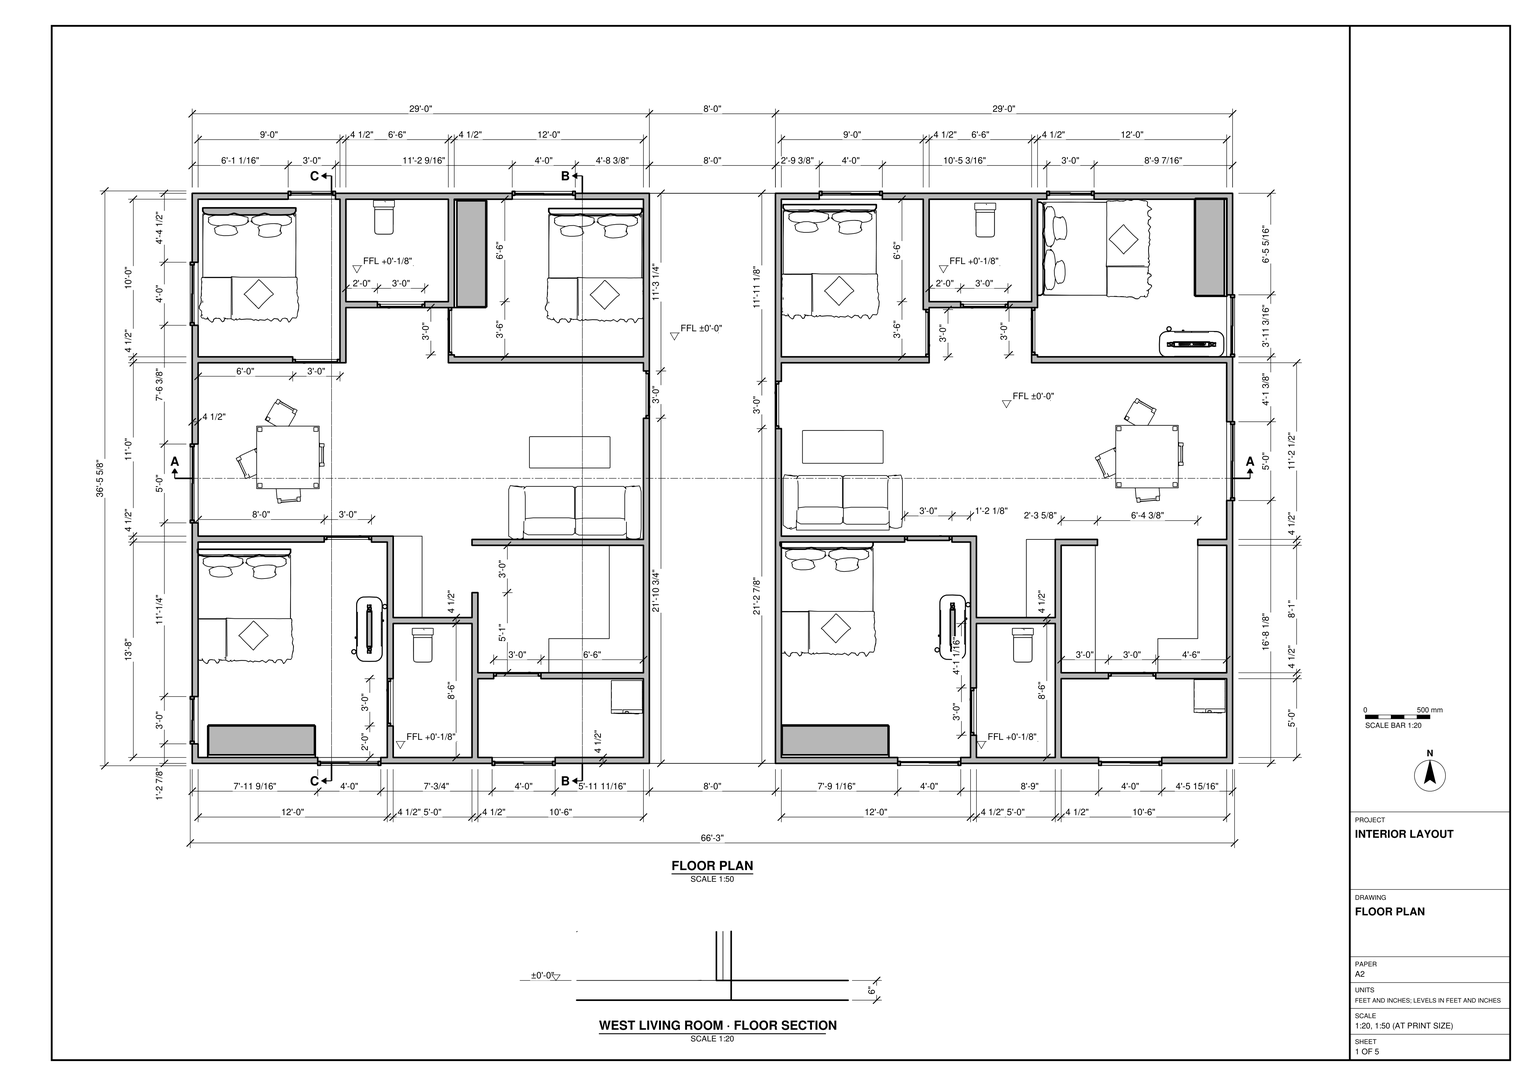
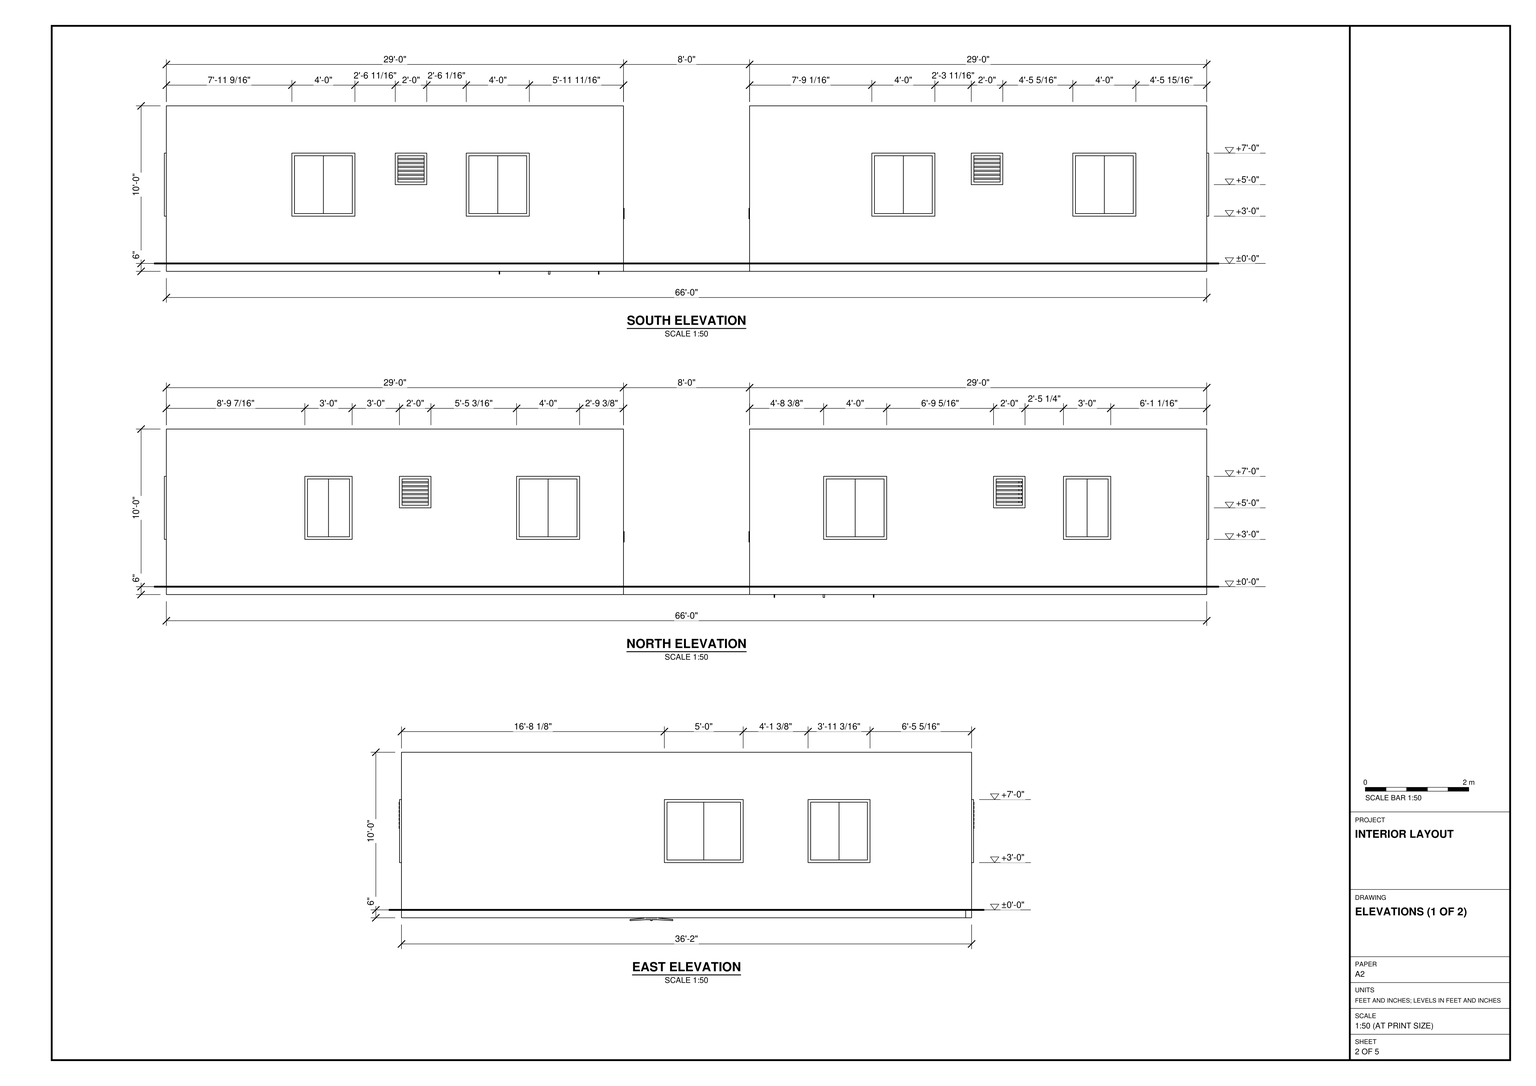
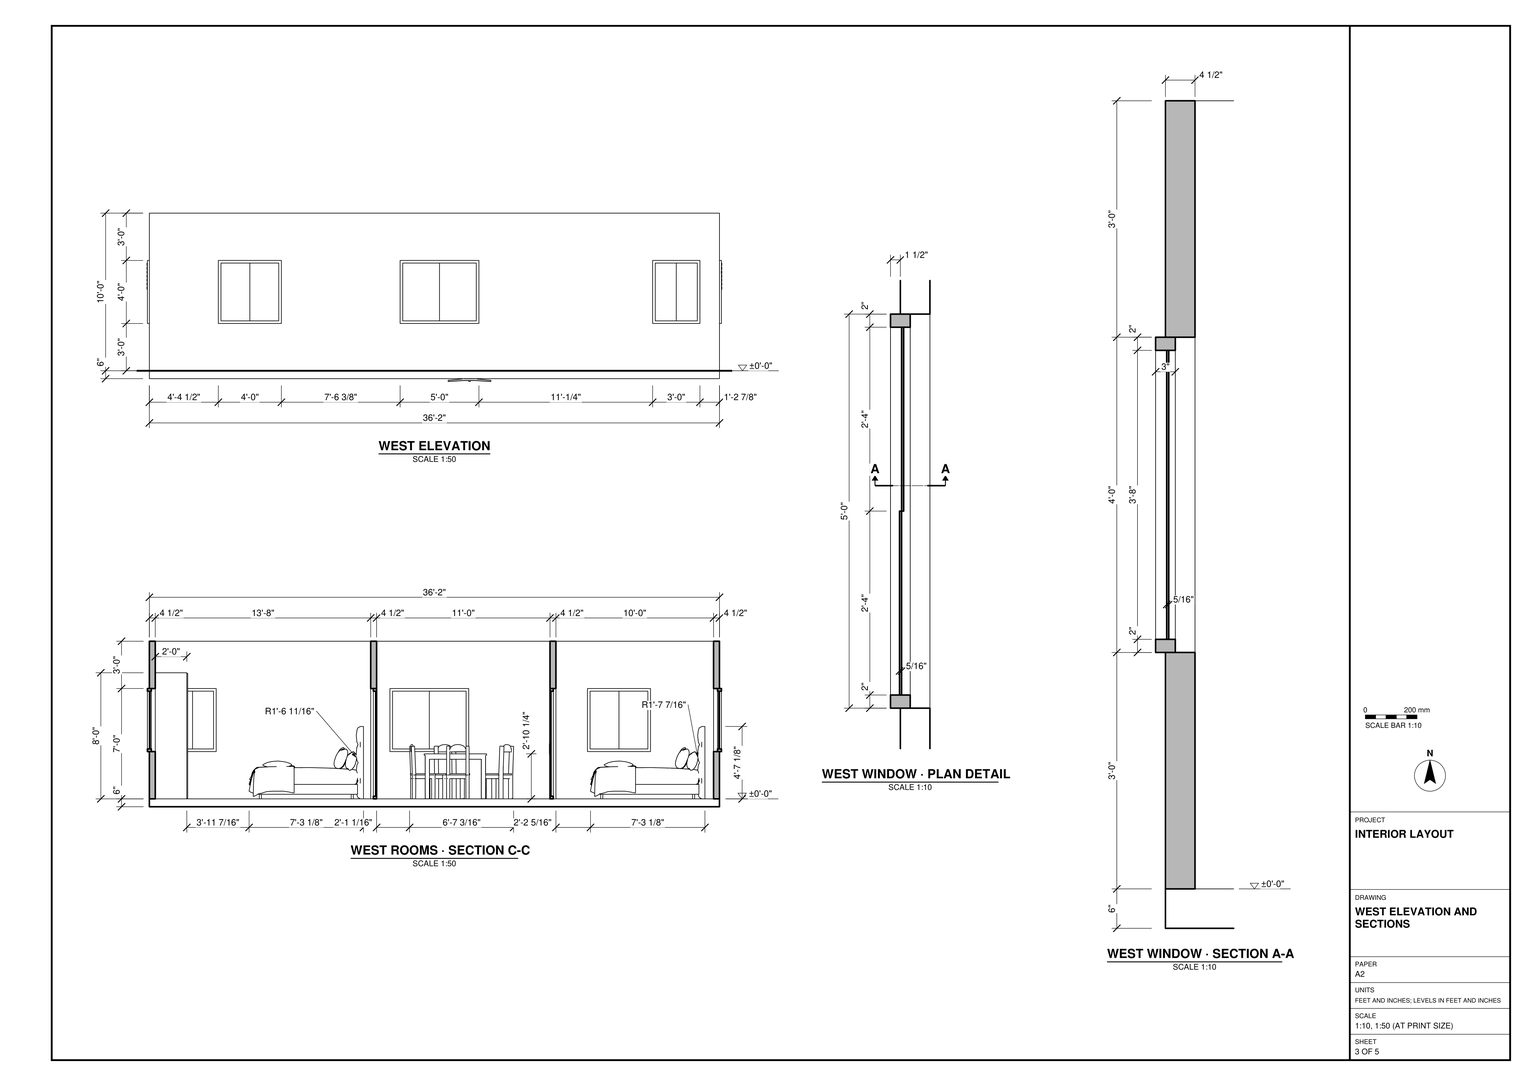
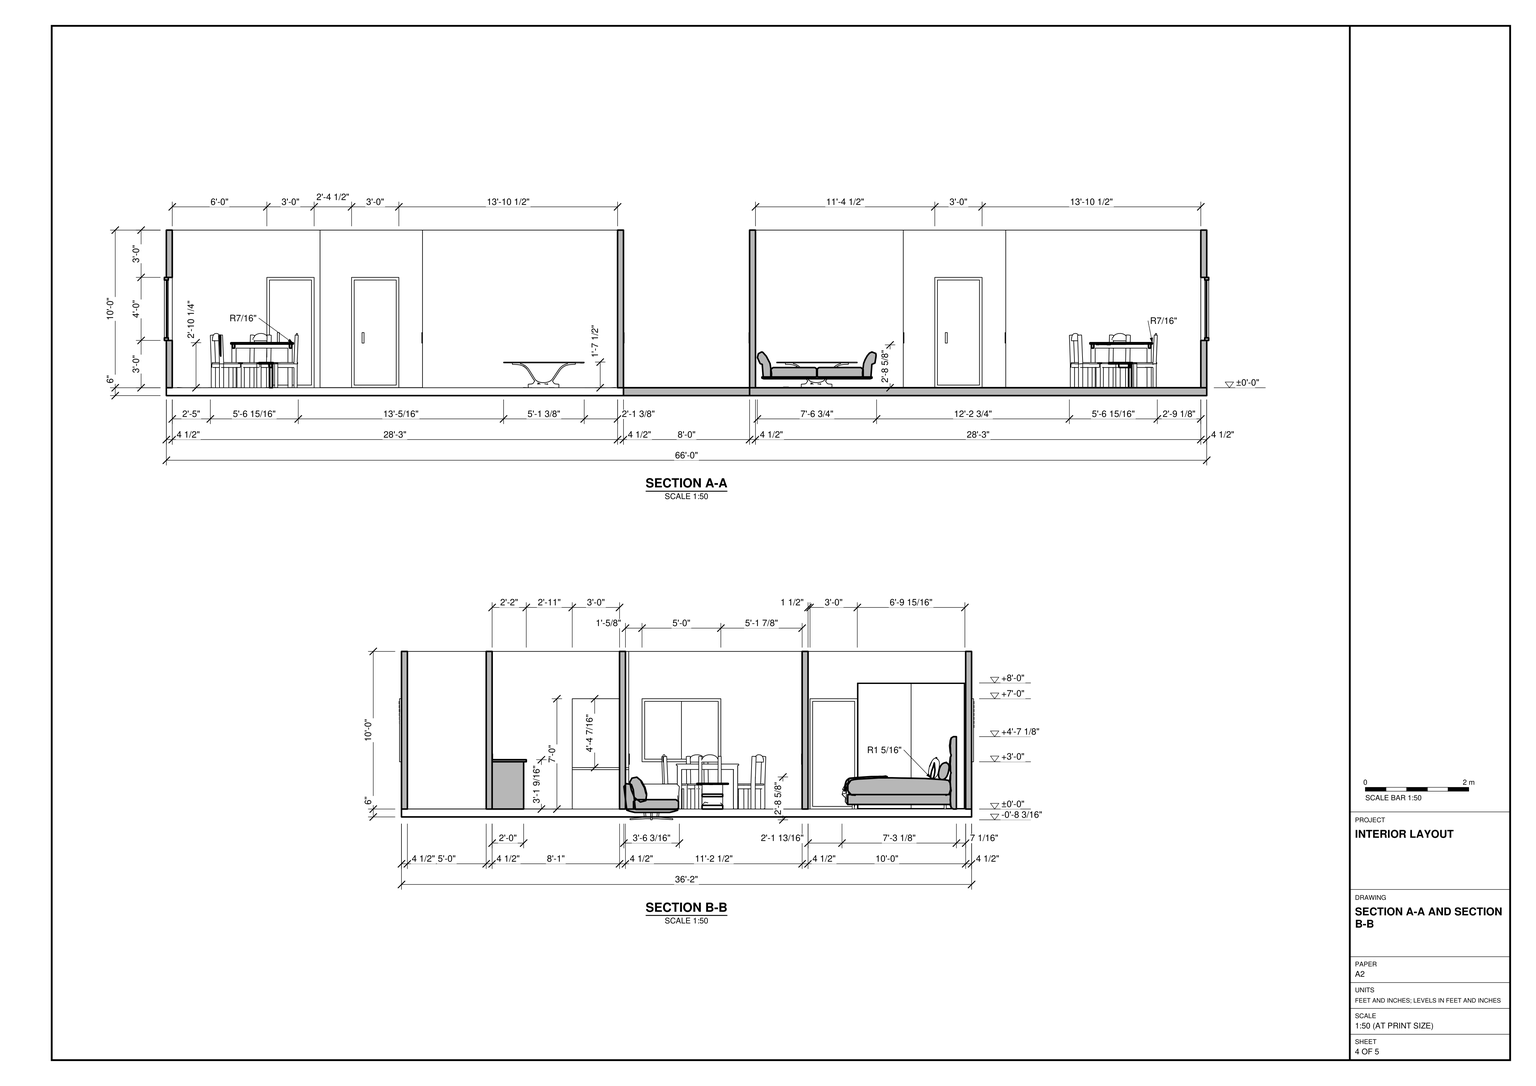
Build both single-storey interiors in SketchUp from task_files/diagram_01.pdf. Work in feet and inches. The overall model measures 66'-3" east to west, 36'-5 5/8" north to south and 10'-8 3/16" high. Use ±0'-0" as the ground-floor level. Set the two 29'-0" wide enclosures side by side with an 8'-0" clear gap between their facing walls.

Model the floor slab, the 4 1/2" walls and the doorways at the positions shown in plan. Use the elevations and window details to set out the glazed openings, frames and louvred vents. In each interior, arrange the northern bedrooms around the small toilet room. Reproduce the southern bedroom, toilet room and service spaces, including their staggered partitions and joinery.

Keep the central living and dining areas open. Place each sofa and low table toward the gap and each dining set toward the outer wall. Follow the plan for bed orientations, storage positions, fixtures and appliances, and use the sections to size the furniture and tall storage. Decor and loose items, including appliances, may be any suitable library components.

Keep shell elements and individual furniture and joinery pieces in separate groups or components, and use components for repeated parts. Save one SketchUp model as output_files/two_furnished_residential_interiors_side_by_side.skp.

# SketchUp Ruby script. Lengths in inches.
U = 1.inch
M = Sketchup.active_model
def pt(a) = Geom::Point3d.new(a.map { |v| v * U })
def face(e, loops, mat)
  f = e.add_face(loops[0].map { |a| pt(a) })
  loops[1..].each { |l| e.add_face(l.map { |a| pt(a) }).erase! }
  f.material = f.back_material = mat if mat
  f
end
# faces: each face lists its corners as indices into pts; further lists are holes
def faces(e, pts, list, mat = nil) = list.each { |f| face(e, (f[0].is_a?(Array) ? f : [f]).map { |l| l.map { |i| pts[i] } }, mat) }
# xy, xz, yz: faces in a plane at the given z, y or x. An outline is a flat list of corners, or four numbers for a rectangle; further outlines are holes
def ring(l) = l.size == 4 ? [[l[0], l[1]], [l[2], l[1]], [l[2], l[3]], [l[0], l[3]]] : l.each_slice(2).to_a
def flat(e, list, mat, &to3) = list.each { |f| face(e, (f[0].is_a?(Array) ? f : [f]).map { |l| ring(l).map { |u, v| to3.(u, v) } }, mat) }
def xy(e, z, list, mat = nil) = flat(e, list, mat) { |x, y| [x, y, z] }
def xz(e, y, list, mat = nil) = flat(e, list, mat) { |x, z| [x, y, z] }
def yz(e, x, list, mat = nil) = flat(e, list, mat) { |y, z| [x, y, z] }
def lines(e, pts, list) = list.each { |a, b| e.add_line(pt(pts[a]), pt(pts[b])) }
# prism: a flat outline (further loops are holes) pulled along v
def prism(e, loops, v, mat = nil)
  f = face(e, loops, mat); d = Geom::Vector3d.new(v.map { |x| x * U })
  f.pushpull(f.normal.samedirection?(d) ? d.length : -d.length)
end
def box(e, o, s, mat = nil) = prism(e, [[o, [o[0] + s[0], o[1], o[2]], [o[0] + s[0], o[1] + s[1], o[2]], [o[0], o[1] + s[1], o[2]]]], [0, 0, s[2]], mat)
def at(x, y, z, deg = 0) = Geom::Transformation.translation(pt([x, y, z])) * Geom::Transformation.rotation(ORIGIN, Z_AXIS, deg.degrees)
def axes(o, x, y, z) = Geom::Transformation.new([*x, 0, *y, 0, *z, 0, *pt(o).to_a, 1])
def part(name) = M.definitions.add(name)
# library, detail: a bought-in or finely detailed component or shape, given as its bounding box
def library(name, o, s) = part(name).tap { |d| box(d.entities, o, s) }
def detail(e, o, s) = box(e.add_group.entities, o, s)
def put(e, d, t, mat = nil) = e.add_instance(d, t).tap { |i| i.material = mat if mat }
def group(e, t, mat = nil) = e.add_group.tap { |g| g.transformation = t; g.material = mat if mat }.entities
root = M.entities
M.materials.add("Brown Tiles 240cm").color = [175, 145, 136]
M.materials.add("Glass Opaque Gradient Cubes 240cm").color = [188, 188, 188]
M.materials["Glass Opaque Gradient Cubes 240cm"].alpha = 0.1
M.materials.add("Marble White SSS 100cm").color = [222, 222, 222]
M.materials.add("Metal Sandblasted Black 200cm").color = [86, 90, 95]
M.materials.add("Porcelain Dusk Blue Matte 001").color = [122, 143, 157]
M.materials.add("Tiles Marble Orange 01 160cm").color = [230, 204, 174]
M.materials.add("Two Color Maple Panels 300cm").color = [56, 46, 41]
M.materials.add("Venetian Plaster Black 300cm").color = [50, 50, 50]
c1 = library("Toilet Bowl 127 010",[-8,-12.9,0],[16,25.8,38.91])
c2 = library("Bed 003",[-38.05,-87.1,0],[75.86,87.1,55.12])
c3 = library("Slow",[-50.42,-21.27,0],[100.85,42.21,32.64])
c4 = library("Toy Table Set 40-09",[-39.37,-33.7,0],[66.93,79.21,41.36])
c5 = library("Table 142 031",[-30.7,-14.21,0],[61.4,28.42,19.53])
c6 = library("Ballet 2 Collar",[-24.63,-13.64,0],[49.35,27.27,70])
c7 = library("Washer 001",[-11.8125,-12.73,0],[23.63,25.47,33.9])
c8 = part("Group\#25")
box(c8.entities,[0,0,0],[22,0.31,44])
c9 = part("Group\#27")
box(c9.entities,[0,-0.31,0],[20,0.31,2])
c10 = part("Group\#29")
box(c10.entities,[0,0,0],[22,0.31,44])
c11 = part("Group\#31")
box(c11.entities,[0,0,0],[0.31,16,44])
c12 = part("Group\#33")
box(c12.entities,[0,0,0],[0.31,28,44])
c13 = part("Group\#35")
box(c13.entities,[0,0,0],[0.31,22,44])
c14 = part("Group\#37")
box(c14.entities,[0,-0.31,0],[16,0.31,44])
c15 = part("Group\#39")
box(c15.entities,[0,0,0],[20,0.31,2])
c16 = part("Group\#41")
box(c16.entities,[0,-0.31,0],[22,0.31,44])
c17 = part("Group\#45")
box(c17.entities,[0,-0.31,0],[16,0.31,44])
c18 = part("Group\#47")
box(c18.entities,[0,0,0],[20,0.31,2])
c19 = part("Group\#49")
box(c19.entities,[0,-0.31,0],[22,0.31,44])
c20 = part("Group\#53")
box(c20.entities,[-0.31,0,0],[0.31,28,44])
c21 = part("Group\#55")
box(c21.entities,[0,0,0],[22,0.31,44])
c22 = part("Group\#92")
box(c22.entities,[0,-0.31,0],[20,0.31,2])
c23 = part("Group\#59")
box(c23.entities,[0,0,0],[22,0.31,44])
c24 = part("Group\#51")
box(c24.entities,[-0.31,0,0],[0.31,21.59,44])
c25 = part("Group\#91")
box(c25.entities,[0,0,0],[40.32,0.71,118.74])
c26 = part("Group\#90")
xy(c26.entities,0,[[0,0,81.91,24]])
xy(c26.entities,0.63,[[0.63,2,81.28,24]])
xy(c26.entities,119.37,[[0.63,2,81.28,24]])
xy(c26.entities,120,[[0,0,81.91,24]])
xz(c26.entities,0,[[0,0,81.91,120]])
xz(c26.entities,2,[[0.63,0.63,81.28,119.37]])
xz(c26.entities,24,[[[0.1,0.1,81.81,119.9],[0.63,0.63,81.28,119.37]]])
yz(c26.entities,0,[[0,0,24,120]])
yz(c26.entities,0.63,[[2,0.63,24,119.37]])
yz(c26.entities,81.28,[[2,0.63,24,119.37]])
yz(c26.entities,81.91,[[0,0,24,120]])
put(c26.entities,c25,at(40.95,24,0.63))
put(c26.entities,c25,at(0.63,24,0.63))
xy(root,-6,[[1.5,1.81,349.5,435.81]],"Marble White SSS 100cm")
xy(root,-0.1,[[562.5,353.31,640.5,431.31]])
xy(root,0,[[598.5,6.31,658.5,108.31]])
xy(root,0,[[154.5,6.31,214.5,108.31],[118.5,353.31,196.5,431.31]],"Brown Tiles 240cm")
xy(root,0.1,[[154.5,6.31,214.5,108.31],[598.5,6.31,658.5,108.31],[118.5,353.31,196.5,431.31],[562.5,353.31,640.5,431.31]],"Tiles Marble Orange 01 160cm")
xz(root,6.31,[[598.5,0,658.5,0.1]])
xz(root,6.31,[[154.5,0,214.5,0.1]],"Brown Tiles 240cm")
xz(root,108.31,[[598.5,0,658.5,0.1]])
xz(root,108.31,[[154.5,0,214.5,0.1]],"Brown Tiles 240cm")
xz(root,353.31,[[562.5,-0.1,640.5,0.1]])
xz(root,353.31,[[118.5,0,196.5,0.1]],"Brown Tiles 240cm")
xz(root,431.31,[[562.5,-0.1,640.5,0.1]])
xz(root,431.31,[[118.5,0,196.5,0.1]],"Brown Tiles 240cm")
yz(root,118.5,[[353.31,0,431.31,0.1]],"Brown Tiles 240cm")
yz(root,154.5,[[6.31,0,108.31,0.1]],"Brown Tiles 240cm")
yz(root,196.5,[[353.31,0,431.31,0.1]],"Brown Tiles 240cm")
yz(root,214.5,[[6.31,0,108.31,0.1]],"Brown Tiles 240cm")
yz(root,562.5,[[353.31,-0.1,431.31,0.1]])
yz(root,598.5,[[6.31,0,108.31,0.1]])
yz(root,640.5,[[353.31,-0.1,431.31,0.1]])
yz(root,658.5,[[6.31,0,108.31,0.1]])
put(root,c1,at(147.47,417.55,0))
put(root,c1,at(605.2,415.45,0))
put(root,c1,at(177.01,91.76,0))
put(root,c1,at(633.82,91.76,0))
put(root,c2,at(486.74,427.2,0))
put(root,c2,at(644.88,393.51,0,90))
put(root,c2,at(308.29,424.24,0))
put(root,c2,at(44.87,424.73,0))
put(root,c2,at(40.86,164.82,0))
put(root,c2,at(484.29,170.31,0))
put(root,c3,at(292.86,192.07,-8.2,-180))
put(root,c4,at(74.35,233.6,0))
put(root,c4,at(728.32,234.2,0))
put(root,c3,axes([496.8,200.35,0],[-0.9,0,0],[0,-1,0],[0,0,1]))
put(root,c5,axes([496.77,242.77,0],[1,0,0],[0,0.88,0],[0,0,1]))
put(root,c5,axes([288.91,238.64,0],[1,0,0],[0,0.84,0],[0,0,1]))
put(root,c6,at(762.26,320.84,0))
put(root,c6,at(136.37,104.05,0,-90))
put(root,c6,at(580.37,105.51,0,-90))
put(root,c7,at(775.96,52.82,0))
put(root,c7,at(332.35,52.17,0))
g1 = group(root,at(102,174.81,0))
prism(g1,[[[36,0,0],[0,0,0],[0,0,84],[36,0,84]],[[2,0,82],[2,0,2],[34,0,2],[34,0,82]]],[0,-2.5,0],"Metal Sandblasted Black 200cm")
g2 = group(g1,at(2,0,2))
box(g2,[0,-0.71,0],[32,0.71,80],"Two Color Maple Panels 300cm")
g3 = group(g2,at(26,0,32),"Metal Sandblasted Black 200cm")
box(g3,[-1.5,0,0],[1.5,0.5,8])
g4 = group(root,at(1.5,-55.69,0))
xy(g4,0,[[0,57.5,0,491.5,348,491.5,348,356.25,343.5,356.25,343.5,362.5,195,362.5,195,368.5,199.5,368.5,199.5,367,343.5,367,343.5,487,199.5,487,199.5,404.5,177,404.5,177,409,195,409,195,487,117,487,117,409,141,409,141,404.5,117,404.5,117,362.5,112.5,362.5,112.5,487,4.5,487,4.5,367,76.5,367,76.5,362.5,4.5,362.5,4.5,230.5,100.5,230.5,100.5,226,4.5,226,4.5,62,148.5,62,148.5,86,153,86,153,62,213,62,213,164,153,164,153,122,148.5,122,148.5,226,136.5,226,136.5,230.5,153,230.5,153,168.5,213,168.5,213,187.5,217.5,187.5,217.5,126.5,229.5,126.5,229.5,122,217.5,122,217.5,62,343.5,62,343.5,122,265.5,122,265.5,126.5,343.5,126.5,343.5,223.5,213,223.5,213,228,343.5,228,343.5,320.25,348,320.25,348,57.5]],"Porcelain Dusk Blue Matte 001")
xy(g4,36,[[95.5625,57.5,143.5625,62],[228.3125,57.5,276.3125,62],[0,72.375,4.5,108.375],[0,240.625,4.5,300.625],[0,391,4.5,439],
  [73.0625,487,109.0625,491.5],[243.625,487,291.625,491.5]],"Porcelain Dusk Blue Matte 001")
xy(g4,60,[[174.25,57.5,198.25,62],[138.3125,487,162.3125,491.5]],"Porcelain Dusk Blue Matte 001")
xy(g4,84,[[95.5625,57.5,143.5625,62],[174.25,57.5,198.25,62],[228.3125,57.5,276.3125,62],[0,72.375,4.5,108.375],[148.5,86,153,122],
  [229.5,122,265.5,126.5],[213,187.5,217.5,223.5],[100.5,226,136.5,230.5],[0,240.625,4.5,300.625],[343.5,320.25,348,356.25],
  [76.5,362.5,112.5,367],[195,368.5,199.5,404.5],[0,391,4.5,439],[141,404.5,177,409],[73.0625,487,109.0625,491.5],
  [138.3125,487,162.3125,491.5],[243.625,487,291.625,491.5]],"Porcelain Dusk Blue Matte 001")
xy(g4,120,[[[0,57.5,348,491.5],[153,168.5,153,230.5,4.5,230.5,4.5,362.5,117,362.5,117,404.5,195,404.5,195,362.5,343.5,362.5,343.5,228,213,228,213,168.5],[4.5,62,148.5,226],[199.5,367,343.5,487],[4.5,367,112.5,487],[217.5,126.5,343.5,223.5],[217.5,62,343.5,122],[153,62,213,164],[117,409,195,487]]],"Porcelain Dusk Blue Matte 001")
xz(g4,57.5,[[[0,0,348,120],[95.5625,36,143.5625,84],[228.3125,36,276.3125,84],[174.25,60,198.25,84]]],"Porcelain Dusk Blue Matte 001")
xz(g4,62,[[[4.5,0,148.5,120],[95.5625,36,143.5625,84]],[[153,0,213,120],[174.25,60,198.25,84]],[[217.5,0,343.5,120],[228.3125,36,276.3125,84]]],"Porcelain Dusk Blue Matte 001")
xz(g4,72.375,[[0,36,4.5,84]],"Porcelain Dusk Blue Matte 001")
xz(g4,86,[[148.5,0,153,84]],"Porcelain Dusk Blue Matte 001")
xz(g4,108.375,[[0,36,4.5,84]],"Porcelain Dusk Blue Matte 001")
xz(g4,122,[[148.5,0,153,84],[217.5,0,229.5,0,229.5,84,265.5,84,265.5,0,343.5,0,343.5,120,217.5,120]],"Porcelain Dusk Blue Matte 001")
xz(g4,126.5,[[217.5,0,217.5,120,343.5,120,343.5,0,265.5,0,265.5,84,229.5,84,229.5,0]],"Porcelain Dusk Blue Matte 001")
xz(g4,164,[[153,0,213,120]],"Porcelain Dusk Blue Matte 001")
xz(g4,168.5,[[153,0,213,120]],"Porcelain Dusk Blue Matte 001")
xz(g4,187.5,[[213,0,217.5,84]],"Porcelain Dusk Blue Matte 001")
xz(g4,223.5,[[213,0,343.5,0,343.5,120,217.5,120,217.5,84,213,84]],"Porcelain Dusk Blue Matte 001")
xz(g4,226,[[4.5,0,100.5,0,100.5,84,136.5,84,136.5,0,148.5,0,148.5,120,4.5,120]],"Porcelain Dusk Blue Matte 001")
xz(g4,228,[[213,0,343.5,120]],"Porcelain Dusk Blue Matte 001")
xz(g4,230.5,[[4.5,0,4.5,120,153,120,153,0,136.5,0,136.5,84,100.5,84,100.5,0]],"Porcelain Dusk Blue Matte 001")
xz(g4,240.625,[[0,36,4.5,84]],"Porcelain Dusk Blue Matte 001")
xz(g4,300.625,[[0,36,4.5,84]],"Porcelain Dusk Blue Matte 001")
xz(g4,320.25,[[343.5,0,348,84]],"Porcelain Dusk Blue Matte 001")
xz(g4,356.25,[[343.5,0,348,84]],"Porcelain Dusk Blue Matte 001")
xz(g4,362.5,[[4.5,0,76.5,0,76.5,84,112.5,84,112.5,0,117,0,117,120,4.5,120],[195,0,343.5,120]],"Porcelain Dusk Blue Matte 001")
xz(g4,367,[[4.5,0,4.5,120,112.5,120,112.5,84,76.5,84,76.5,0],[199.5,0,343.5,120]],"Porcelain Dusk Blue Matte 001")
xz(g4,368.5,[[195,0,199.5,84]],"Porcelain Dusk Blue Matte 001")
xz(g4,391,[[0,36,4.5,84]],"Porcelain Dusk Blue Matte 001")
xz(g4,404.5,[[117,0,141,0,141,84,177,84,177,0,199.5,0,199.5,84,195,84,195,120,117,120]],"Porcelain Dusk Blue Matte 001")
xz(g4,409,[[117,0,117,120,195,120,195,0,177,0,177,84,141,84,141,0]],"Porcelain Dusk Blue Matte 001")
xz(g4,439,[[0,36,4.5,84]],"Porcelain Dusk Blue Matte 001")
xz(g4,487,[[[4.5,0,112.5,120],[73.0625,36,109.0625,84]],[[117,0,195,120],[138.3125,60,162.3125,84]],[[199.5,0,343.5,120],[243.625,36,291.625,84]]],"Porcelain Dusk Blue Matte 001")
xz(g4,491.5,[[[0,0,348,120],[243.625,36,291.625,84],[73.0625,36,109.0625,84],[138.3125,60,162.3125,84]]],"Porcelain Dusk Blue Matte 001")
yz(g4,0,[[[57.5,0,491.5,120],[240.625,36,300.625,84],[391,36,439,84],[72.375,36,108.375,84]]],"Porcelain Dusk Blue Matte 001")
yz(g4,4.5,[[[62,0,226,120],[72.375,36,108.375,84]],[[230.5,0,362.5,120],[240.625,36,300.625,84]],[[367,0,487,120],[391,36,439,84]]],"Porcelain Dusk Blue Matte 001")
yz(g4,73.0625,[[487,36,491.5,84]],"Porcelain Dusk Blue Matte 001")
yz(g4,76.5,[[362.5,0,367,84]],"Porcelain Dusk Blue Matte 001")
yz(g4,95.5625,[[57.5,36,62,84]],"Porcelain Dusk Blue Matte 001")
yz(g4,100.5,[[226,0,230.5,84]],"Porcelain Dusk Blue Matte 001")
yz(g4,109.0625,[[487,36,491.5,84]],"Porcelain Dusk Blue Matte 001")
yz(g4,112.5,[[362.5,0,362.5,84,367,84,367,120,487,120,487,0]],"Porcelain Dusk Blue Matte 001")
yz(g4,117,[[362.5,0,404.5,120],[409,0,487,120]],"Porcelain Dusk Blue Matte 001")
yz(g4,136.5,[[226,0,230.5,84]],"Porcelain Dusk Blue Matte 001")
yz(g4,138.3125,[[487,60,491.5,84]],"Porcelain Dusk Blue Matte 001")
yz(g4,141,[[404.5,0,409,84]],"Porcelain Dusk Blue Matte 001")
yz(g4,143.5625,[[57.5,36,62,84]],"Porcelain Dusk Blue Matte 001")
yz(g4,148.5,[[62,0,62,120,226,120,226,0,122,0,122,84,86,84,86,0]],"Porcelain Dusk Blue Matte 001")
yz(g4,153,[[62,0,86,0,86,84,122,84,122,0,164,0,164,120,62,120],[168.5,0,230.5,120]],"Porcelain Dusk Blue Matte 001")
yz(g4,162.3125,[[487,60,491.5,84]],"Porcelain Dusk Blue Matte 001")
yz(g4,174.25,[[57.5,60,62,84]],"Porcelain Dusk Blue Matte 001")
yz(g4,177,[[404.5,0,409,84]],"Porcelain Dusk Blue Matte 001")
yz(g4,195,[[362.5,0,362.5,120,404.5,120,404.5,84,368.5,84,368.5,0],[409,0,487,120]],"Porcelain Dusk Blue Matte 001")
yz(g4,198.25,[[57.5,60,62,84]],"Porcelain Dusk Blue Matte 001")
yz(g4,199.5,[[367,0,368.5,0,368.5,84,404.5,84,404.5,0,487,0,487,120,367,120]],"Porcelain Dusk Blue Matte 001")
yz(g4,213,[[62,0,164,120],[168.5,0,168.5,120,228,120,228,0,223.5,0,223.5,84,187.5,84,187.5,0]],"Porcelain Dusk Blue Matte 001")
yz(g4,217.5,[[62,0,122,120],[126.5,0,187.5,0,187.5,84,223.5,84,223.5,120,126.5,120]],"Porcelain Dusk Blue Matte 001")
yz(g4,228.3125,[[57.5,36,62,84]],"Porcelain Dusk Blue Matte 001")
yz(g4,229.5,[[122,0,126.5,84]],"Porcelain Dusk Blue Matte 001")
yz(g4,243.625,[[487,36,491.5,84]],"Porcelain Dusk Blue Matte 001")
yz(g4,265.5,[[122,0,126.5,84]],"Porcelain Dusk Blue Matte 001")
yz(g4,276.3125,[[57.5,36,62,84]],"Porcelain Dusk Blue Matte 001")
yz(g4,291.625,[[487,36,491.5,84]],"Porcelain Dusk Blue Matte 001")
yz(g4,343.5,[[62,0,122,120],[126.5,0,223.5,120],[228,0,228,120,362.5,120,362.5,0,356.25,0,356.25,84,320.25,84,320.25,0],[367,0,487,120]],"Porcelain Dusk Blue Matte 001")
yz(g4,348,[[57.5,0,320.25,0,320.25,84,356.25,84,356.25,0,491.5,0,491.5,120,57.5,120]],"Porcelain Dusk Blue Matte 001")
p = [[265.5,126.5,0],[229.5,126.5,0]]
lines(g4,p,[[0,1]])
g5 = group(g4,at(348,320.25,0))
prism(g5,[[[0,36,0],[0,36,84],[0,0,84],[0,0,0]],[[0,2,82],[0,34,82],[0,34,2],[0,2,2]]],[-2.5,0,0],"Metal Sandblasted Black 200cm")
g6 = group(g5,at(0,2,2))
box(g6,[-0.71,0,0],[0.71,32,80],"Two Color Maple Panels 300cm")
g7 = group(g6,at(0,6,32),"Metal Sandblasted Black 200cm")
box(g7,[0,0,0],[0.5,1.5,8])
g8 = group(g4,at(148.5,86,0))
prism(g8,[[[0,0,0],[0,0,84],[0,36,84],[0,36,0]],[[0,2,2],[0,34,2],[0,34,82],[0,2,82]]],[2.5,0,0],"Metal Sandblasted Black 200cm")
g9 = group(g8,at(0,2,2))
box(g9,[0,0,0],[0.71,32,80],"Two Color Maple Panels 300cm")
g10 = group(g9,at(0,26,32),"Metal Sandblasted Black 200cm")
box(g10,[-0.5,-1.5,0],[0.5,1.5,8])
g11 = group(g4,at(76.5,362.5,0))
prism(g11,[[[36,0,0],[36,0,84],[0,0,84],[0,0,0]],[[2,0,2],[2,0,82],[34,0,82],[34,0,2]]],[0,2.5,0],"Metal Sandblasted Black 200cm")
g12 = group(g11,at(2,0,2))
box(g12,[0,0,0],[32,0.71,80],"Two Color Maple Panels 300cm")
g13 = group(g12,at(6,0,32),"Metal Sandblasted Black 200cm")
box(g13,[0,-0.5,0],[1.5,0.5,8])
g14 = group(g4,at(141,404.5,0))
prism(g14,[[[36,0,0],[36,0,84],[0,0,84],[0,0,0]],[[34,0,2],[2,0,2],[2,0,82],[34,0,82]]],[0,2.5,0],"Metal Sandblasted Black 200cm")
g15 = group(g14,at(2,0,2))
box(g15,[0,0,0],[32,0.71,80],"Two Color Maple Panels 300cm")
g16 = group(g15,at(6,0,32),"Metal Sandblasted Black 200cm")
box(g16,[0,-0.5,0],[1.5,0.5,8])
g17 = group(g4,at(195,368.5,0))
prism(g17,[[[0,0,0],[0,0,84],[0,36,84],[0,36,0]],[[0,34,2],[0,34,82],[0,2,82],[0,2,2]]],[2.5,0,0],"Metal Sandblasted Black 200cm")
g18 = group(g17,at(0,2,2))
box(g18,[0,0,0],[0.71,32,80],"Two Color Maple Panels 300cm")
g19 = group(g18,at(0,26,32),"Metal Sandblasted Black 200cm")
box(g19,[-0.5,-1.5,0],[0.5,1.5,8])
g20 = group(g4,at(95.5625,57.5,36))
prism(g20,[[[48,-1.5,0],[48,-1.5,48],[0,-1.5,48],[0,-1.5,0]],[[2,-1.5,2],[2,-1.5,46],[46,-1.5,46],[46,-1.5,2]]],[0,3,0],"Metal Sandblasted Black 200cm")
put(g20,c8,at(2,0.125,2),"Glass Opaque Gradient Cubes 240cm")
put(g20,c8,at(24,-0.19,2),"Glass Opaque Gradient Cubes 240cm")
g21 = group(g4,at(174.25,57.5,60))
prism(g21,[[[0,-1.5,0],[24,-1.5,0],[24,-1.5,24],[0,-1.5,24]],[[2,-1.5,22],[22,-1.5,22],[22,-1.5,2],[2,-1.5,2]]],[0,3,0],"Metal Sandblasted Black 200cm")
put(g21,c9,at(2,-1.5,20),"Glass Opaque Gradient Cubes 240cm")
put(g21,c9,at(2,-1.45,17),"Glass Opaque Gradient Cubes 240cm")
put(g21,c9,at(2,-1.4,14),"Glass Opaque Gradient Cubes 240cm")
put(g21,c9,at(2,-1.34,11),"Glass Opaque Gradient Cubes 240cm")
put(g21,c9,at(2,-1.29,8),"Glass Opaque Gradient Cubes 240cm")
put(g21,c9,at(2,-1.24,5),"Glass Opaque Gradient Cubes 240cm")
put(g21,c9,at(2,-1.19,2),"Glass Opaque Gradient Cubes 240cm")
g22 = group(g4,at(228.3125,57.5,36))
prism(g22,[[[0,-1.5,0],[48,-1.5,0],[48,-1.5,48],[0,-1.5,48]],[[46,-1.5,2],[2,-1.5,2],[2,-1.5,46],[46,-1.5,46]]],[0,3,0],"Metal Sandblasted Black 200cm")
put(g22,c10,at(2,0.1875,2),"Glass Opaque Gradient Cubes 240cm")
put(g22,c10,at(24,-0.13,2),"Glass Opaque Gradient Cubes 240cm")
g23 = group(g4,at(0,72.375,36))
prism(g23,[[[-1.5,36,0],[-1.5,0,0],[-1.5,0,48],[-1.5,36,48]],[[-1.5,34,2],[-1.5,34,46],[-1.5,2,46],[-1.5,2,2]]],[3,0,0],"Metal Sandblasted Black 200cm")
put(g23,c11,at(0.1875,18,2),"Glass Opaque Gradient Cubes 240cm")
put(g23,c11,at(-0.13,2,2),"Glass Opaque Gradient Cubes 240cm")
g24 = group(g4,at(0,240.625,36))
prism(g24,[[[-1.5,60,0],[-1.5,0,0],[-1.5,0,48],[-1.5,60,48]],[[-1.5,2,2],[-1.5,58,2],[-1.5,58,46],[-1.5,2,46]]],[3,0,0],"Metal Sandblasted Black 200cm")
put(g24,c12,at(0.1875,30,2),"Glass Opaque Gradient Cubes 240cm")
put(g24,c12,at(-0.13,2,2),"Glass Opaque Gradient Cubes 240cm")
g25 = group(g4,at(0,391,36))
prism(g25,[[[-1.5,0,0],[-1.5,0,48],[-1.5,48,48],[-1.5,48,0]],[[-1.5,2,46],[-1.5,2,2],[-1.5,46,2],[-1.5,46,46]]],[3,0,0],"Metal Sandblasted Black 200cm")
put(g25,c13,at(0.0625,24,2),"Glass Opaque Gradient Cubes 240cm")
put(g25,c13,at(-0.25,2,2),"Glass Opaque Gradient Cubes 240cm")
g26 = group(g4,at(73.0625,491.5,36))
prism(g26,[[[0,1.5,0],[0,1.5,48],[36,1.5,48],[36,1.5,0]],[[34,1.5,2],[34,1.5,46],[2,1.5,46],[2,1.5,2]]],[0,-3,0],"Metal Sandblasted Black 200cm")
put(g26,c14,at(18,-0.125,2),"Glass Opaque Gradient Cubes 240cm")
put(g26,c14,at(2,0.19,2),"Glass Opaque Gradient Cubes 240cm")
g27 = group(g4,at(138.3125,491.5,60))
prism(g27,[[[24,1.5,0],[0,1.5,0],[0,1.5,24],[24,1.5,24]],[[2,1.5,2],[22,1.5,2],[22,1.5,22],[2,1.5,22]]],[0,-3,0],"Metal Sandblasted Black 200cm")
put(g27,c15,at(2,1.5,20),"Glass Opaque Gradient Cubes 240cm")
put(g27,c15,at(2,1.5,17),"Glass Opaque Gradient Cubes 240cm")
put(g27,c15,at(2,1.5,14),"Glass Opaque Gradient Cubes 240cm")
put(g27,c15,at(2,1.5,11),"Glass Opaque Gradient Cubes 240cm")
put(g27,c15,at(2,1.5,8),"Glass Opaque Gradient Cubes 240cm")
put(g27,c15,at(2,1.5,5),"Glass Opaque Gradient Cubes 240cm")
put(g27,c15,at(2,1.5,2),"Glass Opaque Gradient Cubes 240cm")
g28 = group(g4,at(243.625,491.5,36))
prism(g28,[[[48,1.5,0],[0,1.5,0],[0,1.5,48],[48,1.5,48]],[[2,1.5,46],[2,1.5,2],[46,1.5,2],[46,1.5,46]]],[0,-3,0],"Metal Sandblasted Black 200cm")
put(g28,c16,at(24,-0.5625,2),"Glass Opaque Gradient Cubes 240cm")
put(g28,c16,at(2,-0.25,2),"Glass Opaque Gradient Cubes 240cm")
g29 = group(g4,at(229.5,126.5,0))
prism(g29,[[[0,0,0],[0,0,84],[36,0,84],[36,0,0]],[[2,0,82],[2,0,2],[34,0,2],[34,0,82]]],[0,-2.5,0],"Metal Sandblasted Black 200cm")
g30 = group(g29,at(2,0,2))
box(g30,[0,-0.71,0],[32,0.71,80],"Two Color Maple Panels 300cm")
g31 = group(g30,at(26,0,32),"Metal Sandblasted Black 200cm")
box(g31,[-1.5,0,0],[1.5,0.5,8])
g32 = group(root,at(154.5,112.81,0))
box(g32,[0,0,0],[20,62,30])
g33 = group(root,at(445.5,1.81,0))
xy(g33,0,[[0,0,0,254.875,4.5,254.875,4.5,173,98.375,173,98.375,168.5,4.5,168.5,4.5,4.5,148.5,4.5,148.5,21.4375,153,21.4375,153,4.5,213,4.5,213,106.5,153,106.5,153,57.4375,148.5,57.4375,148.5,168.5,134.375,168.5,134.375,173,153,173,153,111,213,111,213,170.5,245.125,170.5,245.125,166,217.5,166,217.5,69,253.5,69,253.5,64.5,217.5,64.5,217.5,4.5,343.5,4.5,343.5,64.5,289.5,64.5,289.5,69,343.5,69,343.5,166,321.5,166,321.5,170.5,343.5,170.5,343.5,305,195,305,195,311,199.5,311,199.5,309.5,343.5,309.5,343.5,429.5,199.5,429.5,199.5,347,177,347,177,351.5,195,351.5,195,429.5,117,429.5,117,351.5,141,351.5,141,347,117,347,117,345.5,112.5,345.5,112.5,429.5,4.5,429.5,4.5,309.5,117,309.5,117,305,4.5,305,4.5,290.875,0,290.875,0,434,348,434,348,0],[148.5,21.4375,153,57.4375]],"Porcelain Dusk Blue Matte 001")
xy(g33,36,[[93.0625,0,141.0625,4.5],[246.0625,0,294.0625,4.5],[343.5,200.125,348,260.125],[343.5,309.5,348,356.6875],[33.375,429.5,81.375,434],
  [206.5625,429.5,242.5625,434]],"Porcelain Dusk Blue Matte 001")
xy(g33,60,[[168.75,0,192.75,4.5],[146.5625,429.5,170.5625,434]],"Porcelain Dusk Blue Matte 001")
xy(g33,84,[[93.0625,0,141.0625,4.5],[168.75,0,192.75,4.5],[246.0625,0,294.0625,4.5],[148.5,21.4375,153,57.4375],[253.5,64.5,289.5,69],
  [245.125,166,321.5,170.5],[98.375,168.5,134.375,173],[343.5,200.125,348,260.125],[0,254.875,4.5,290.875],[112.5,309.5,117,345.5],
  [343.5,309.5,348,356.6875],[195,311,199.5,347],[141,347,177,351.5],[33.375,429.5,81.375,434],[146.5625,429.5,170.5625,434],
  [206.5625,429.5,242.5625,434]],"Porcelain Dusk Blue Matte 001")
xy(g33,120,[[[0,0,348,434],[153,111,153,173,4.5,173,4.5,305,117,305,117,347,195,347,195,305,343.5,305,343.5,170.5,213,170.5,213,111],[4.5,4.5,148.5,168.5],[199.5,309.5,343.5,429.5],[4.5,309.5,112.5,429.5],[217.5,69,343.5,166],[217.5,4.5,343.5,64.5],[153,4.5,213,106.5],[117,351.5,195,429.5]]],"Porcelain Dusk Blue Matte 001")
xz(g33,0,[[[0,0,348,120],[93.0625,36,141.0625,84],[246.0625,36,294.0625,84],[168.75,60,192.75,84]]],"Porcelain Dusk Blue Matte 001")
xz(g33,4.5,[[[4.5,0,148.5,120],[93.0625,36,141.0625,84]],[[153,0,213,120],[168.75,60,192.75,84]],[[217.5,0,343.5,120],[246.0625,36,294.0625,84]]],"Porcelain Dusk Blue Matte 001")
xz(g33,21.4375,[[148.5,0,153,84]],"Porcelain Dusk Blue Matte 001")
xz(g33,57.4375,[[148.5,0,153,84]],"Porcelain Dusk Blue Matte 001")
xz(g33,64.5,[[217.5,0,253.5,0,253.5,84,289.5,84,289.5,0,343.5,0,343.5,120,217.5,120]],"Porcelain Dusk Blue Matte 001")
xz(g33,69,[[217.5,0,217.5,120,343.5,120,343.5,0,289.5,0,289.5,84,253.5,84,253.5,0]],"Porcelain Dusk Blue Matte 001")
xz(g33,106.5,[[153,0,213,120]],"Porcelain Dusk Blue Matte 001")
xz(g33,111,[[153,0,213,120]],"Porcelain Dusk Blue Matte 001")
xz(g33,166,[[217.5,0,245.125,0,245.125,84,321.5,84,321.5,0,343.5,0,343.5,120,217.5,120]],"Porcelain Dusk Blue Matte 001")
xz(g33,168.5,[[4.5,0,98.375,0,98.375,84,134.375,84,134.375,0,148.5,0,148.5,120,4.5,120]],"Porcelain Dusk Blue Matte 001")
xz(g33,170.5,[[213,0,213,120,343.5,120,343.5,0,321.5,0,321.5,84,245.125,84,245.125,0]],"Porcelain Dusk Blue Matte 001")
xz(g33,173,[[4.5,0,4.5,120,153,120,153,0,134.375,0,134.375,84,98.375,84,98.375,0]],"Porcelain Dusk Blue Matte 001")
xz(g33,200.125,[[343.5,36,348,84]],"Porcelain Dusk Blue Matte 001")
xz(g33,254.875,[[0,0,4.5,84]],"Porcelain Dusk Blue Matte 001")
xz(g33,260.125,[[343.5,36,348,84]],"Porcelain Dusk Blue Matte 001")
xz(g33,290.875,[[0,0,4.5,84]],"Porcelain Dusk Blue Matte 001")
xz(g33,305,[[4.5,0,117,120],[195,0,343.5,120]],"Porcelain Dusk Blue Matte 001")
xz(g33,309.5,[[4.5,0,4.5,120,112.5,120,112.5,84,117,84,117,0],[199.5,0,343.5,120],[343.5,36,348,84]],"Porcelain Dusk Blue Matte 001")
xz(g33,311,[[195,0,199.5,84]],"Porcelain Dusk Blue Matte 001")
xz(g33,345.5,[[112.5,0,117,84]],"Porcelain Dusk Blue Matte 001")
xz(g33,347,[[117,0,141,0,141,84,177,84,177,0,199.5,0,199.5,84,195,84,195,120,117,120]],"Porcelain Dusk Blue Matte 001")
xz(g33,351.5,[[117,0,117,120,195,120,195,0,177,0,177,84,141,84,141,0]],"Porcelain Dusk Blue Matte 001")
xz(g33,356.6875,[[343.5,36,348,84]],"Porcelain Dusk Blue Matte 001")
xz(g33,429.5,[[[4.5,0,112.5,120],[33.375,36,81.375,84]],[[117,0,195,120],[146.5625,60,170.5625,84]],[[199.5,0,343.5,120],[206.5625,36,242.5625,84]]],"Porcelain Dusk Blue Matte 001")
xz(g33,434,[[[0,0,348,120],[33.375,36,81.375,84],[206.5625,36,242.5625,84],[146.5625,60,170.5625,84]]],"Porcelain Dusk Blue Matte 001")
yz(g33,0,[[0,0,0,120,434,120,434,0,290.875,0,290.875,84,254.875,84,254.875,0]],"Porcelain Dusk Blue Matte 001")
yz(g33,4.5,[[4.5,0,168.5,120],[173,0,254.875,0,254.875,84,290.875,84,290.875,0,305,0,305,120,173,120],[309.5,0,429.5,120]],"Porcelain Dusk Blue Matte 001")
yz(g33,33.375,[[429.5,36,434,84]],"Porcelain Dusk Blue Matte 001")
yz(g33,81.375,[[429.5,36,434,84]],"Porcelain Dusk Blue Matte 001")
yz(g33,93.0625,[[0,36,4.5,84]],"Porcelain Dusk Blue Matte 001")
yz(g33,98.375,[[168.5,0,173,84]],"Porcelain Dusk Blue Matte 001")
yz(g33,112.5,[[345.5,0,345.5,84,309.5,84,309.5,120,429.5,120,429.5,0]],"Porcelain Dusk Blue Matte 001")
yz(g33,117,[[305,0,309.5,0,309.5,84,345.5,84,345.5,0,347,0,347,120,305,120],[351.5,0,429.5,120]],"Porcelain Dusk Blue Matte 001")
yz(g33,134.375,[[168.5,0,173,84]],"Porcelain Dusk Blue Matte 001")
yz(g33,141,[[347,0,351.5,84]],"Porcelain Dusk Blue Matte 001")
yz(g33,141.0625,[[0,36,4.5,84]],"Porcelain Dusk Blue Matte 001")
yz(g33,146.5625,[[429.5,60,434,84]],"Porcelain Dusk Blue Matte 001")
yz(g33,148.5,[[4.5,0,4.5,120,168.5,120,168.5,0,57.4375,0,57.4375,84,21.4375,84,21.4375,0]],"Porcelain Dusk Blue Matte 001")
yz(g33,153,[[4.5,0,21.4375,0,21.4375,84,57.4375,84,57.4375,0,106.5,0,106.5,120,4.5,120],[111,0,173,120]],"Porcelain Dusk Blue Matte 001")
yz(g33,168.75,[[0,60,4.5,84]],"Porcelain Dusk Blue Matte 001")
yz(g33,170.5625,[[429.5,60,434,84]],"Porcelain Dusk Blue Matte 001")
yz(g33,177,[[347,0,351.5,84]],"Porcelain Dusk Blue Matte 001")
yz(g33,192.75,[[0,60,4.5,84]],"Porcelain Dusk Blue Matte 001")
yz(g33,195,[[305,0,305,120,347,120,347,84,311,84,311,0],[351.5,0,429.5,120]],"Porcelain Dusk Blue Matte 001")
yz(g33,199.5,[[309.5,0,311,0,311,84,347,84,347,0,429.5,0,429.5,120,309.5,120]],"Porcelain Dusk Blue Matte 001")
yz(g33,206.5625,[[429.5,36,434,84]],"Porcelain Dusk Blue Matte 001")
yz(g33,213,[[4.5,0,106.5,120],[111,0,170.5,120]],"Porcelain Dusk Blue Matte 001")
yz(g33,217.5,[[4.5,0,64.5,120],[69,0,166,120]],"Porcelain Dusk Blue Matte 001")
yz(g33,242.5625,[[429.5,36,434,84]],"Porcelain Dusk Blue Matte 001")
yz(g33,245.125,[[166,0,170.5,84]],"Porcelain Dusk Blue Matte 001")
yz(g33,246.0625,[[0,36,4.5,84]],"Porcelain Dusk Blue Matte 001")
yz(g33,253.5,[[64.5,0,69,84]],"Porcelain Dusk Blue Matte 001")
yz(g33,289.5,[[64.5,0,69,84]],"Porcelain Dusk Blue Matte 001")
yz(g33,294.0625,[[0,36,4.5,84]],"Porcelain Dusk Blue Matte 001")
yz(g33,321.5,[[166,0,170.5,84]],"Porcelain Dusk Blue Matte 001")
yz(g33,343.5,[[4.5,0,64.5,120],[69,0,166,120],[[170.5,0,305,120],[200.125,36,260.125,84]],[309.5,0,309.5,36,356.6875,36,356.6875,84,309.5,84,309.5,120,429.5,120,429.5,0]],"Porcelain Dusk Blue Matte 001")
yz(g33,348,[[[0,0,434,120],[200.125,36,260.125,84],[309.5,36,356.6875,84]]],"Porcelain Dusk Blue Matte 001")
g34 = group(g33,at(193,111,0))
box(g34,[0,0,0],[20,59.5,30])
g35 = group(g33,at(206.5625,434,36))
prism(g35,[[[36,1.5,0],[0,1.5,0],[0,1.5,48],[36,1.5,48]],[[2,1.5,46],[2,1.5,2],[34,1.5,2],[34,1.5,46]]],[0,-3,0],"Metal Sandblasted Black 200cm")
put(g35,c17,at(18,-0.1875,2),"Glass Opaque Gradient Cubes 240cm")
put(g35,c17,at(2,0.13,2),"Glass Opaque Gradient Cubes 240cm")
g36 = group(g33,at(146.5625,434,60))
prism(g36,[[[0,1.5,0],[0,1.5,24],[24,1.5,24],[24,1.5,0]],[[2,1.5,22],[2,1.5,2],[22,1.5,2],[22,1.5,22]]],[0,-3,0],"Metal Sandblasted Black 200cm")
put(g36,c18,at(2,1.5,20),"Glass Opaque Gradient Cubes 240cm")
put(g36,c18,at(2,1.5,17),"Glass Opaque Gradient Cubes 240cm")
put(g36,c18,at(2,1.5,14),"Glass Opaque Gradient Cubes 240cm")
put(g36,c18,at(2,1.5,11),"Glass Opaque Gradient Cubes 240cm")
put(g36,c18,at(2,1.5,8),"Glass Opaque Gradient Cubes 240cm")
put(g36,c18,at(2,1.5,5),"Glass Opaque Gradient Cubes 240cm")
put(g36,c18,at(2,1.5,2),"Glass Opaque Gradient Cubes 240cm")
g37 = group(g33,at(33.375,434,36))
prism(g37,[[[48,1.5,0],[0,1.5,0],[0,1.5,48],[48,1.5,48]],[[2,1.5,2],[46,1.5,2],[46,1.5,46],[2,1.5,46]]],[0,-3,0],"Metal Sandblasted Black 200cm")
put(g37,c19,at(24,-0.3125,2),"Glass Opaque Gradient Cubes 240cm")
put(g37,c19,at(2,0,2),"Glass Opaque Gradient Cubes 240cm")
g38 = group(g33,at(348,200.125,36))
prism(g38,[[[1.5,0,0],[1.5,60,0],[1.5,60,48],[1.5,0,48]],[[1.5,58,46],[1.5,58,2],[1.5,2,2],[1.5,2,46]]],[-3,0,0],"Metal Sandblasted Black 200cm")
put(g38,c20,at(-0.125,2,2),"Glass Opaque Gradient Cubes 240cm")
put(g38,c20,at(0.19,30,2),"Glass Opaque Gradient Cubes 240cm")
g39 = group(g33,at(246.0625,0,36))
prism(g39,[[[0,-1.5,0],[48,-1.5,0],[48,-1.5,48],[0,-1.5,48]],[[46,-1.5,46],[46,-1.5,2],[2,-1.5,2],[2,-1.5,46]]],[0,3,0],"Metal Sandblasted Black 200cm")
put(g39,c21,at(2,0.6875,2),"Glass Opaque Gradient Cubes 240cm")
put(g39,c21,at(24,0.37,2),"Glass Opaque Gradient Cubes 240cm")
g40 = group(g33,at(168.75,0,60))
prism(g40,[[[24,-1.5,0],[24,-1.5,24],[0,-1.5,24],[0,-1.5,0]],[[2,-1.5,22],[22,-1.5,22],[22,-1.5,2],[2,-1.5,2]]],[0,3,0],"Metal Sandblasted Black 200cm")
put(g40,c22,at(2,-1.5,20),"Glass Opaque Gradient Cubes 240cm")
put(g40,c22,at(2,-1.5,17),"Glass Opaque Gradient Cubes 240cm")
put(g40,c22,at(2,-1.5,14),"Glass Opaque Gradient Cubes 240cm")
put(g40,c22,at(2,-1.5,11),"Glass Opaque Gradient Cubes 240cm")
put(g40,c22,at(2,-1.5,8),"Glass Opaque Gradient Cubes 240cm")
g41 = group(g40,at(2,-1.5,5),"Glass Opaque Gradient Cubes 240cm")
box(g41,[0,-0.31,0],[20,0.31,2])
put(g40,c22,at(2,-1.5,2),"Glass Opaque Gradient Cubes 240cm")
g42 = group(g33,at(93.0625,0,36))
prism(g42,[[[48,-1.5,0],[48,-1.5,48],[0,-1.5,48],[0,-1.5,0]],[[46,-1.5,46],[46,-1.5,2],[2,-1.5,2],[2,-1.5,46]]],[0,3,0],"Metal Sandblasted Black 200cm")
put(g42,c23,at(2,0.75,2),"Glass Opaque Gradient Cubes 240cm")
put(g42,c23,at(24,0.44,2),"Glass Opaque Gradient Cubes 240cm")
g43 = group(g33,at(0,254.875,0))
prism(g43,[[[0,36,0],[0,0,0],[0,0,84],[0,36,84]],[[0,2,82],[0,2,2],[0,34,2],[0,34,82]]],[2.5,0,0],"Metal Sandblasted Black 200cm")
g44 = group(g43,at(0,2,2))
box(g44,[0,0,0],[0.71,32,80],"Two Color Maple Panels 300cm")
g45 = group(g44,at(0,26,32),"Metal Sandblasted Black 200cm")
box(g45,[-0.5,-1.5,0],[0.5,1.5,8])
g46 = group(g33,at(117,309.5,0))
prism(g46,[[[0,36,0],[0,36,84],[0,0,84],[0,0,0]],[[0,2,82],[0,34,82],[0,34,2],[0,2,2]]],[-2.5,0,0],"Metal Sandblasted Black 200cm")
g47 = group(g46,at(0,2,2))
box(g47,[-0.71,0,0],[0.71,32,80],"Two Color Maple Panels 300cm")
g48 = group(g47,at(0,6,32),"Metal Sandblasted Black 200cm")
box(g48,[0,0,0],[0.5,1.5,8])
g49 = group(g33,at(141,347,0))
prism(g49,[[[36,0,0],[36,0,84],[0,0,84],[0,0,0]],[[34,0,82],[34,0,2],[2,0,2],[2,0,82]]],[0,2.5,0],"Metal Sandblasted Black 200cm")
g50 = group(g49,at(2,0,2))
box(g50,[0,0,0],[32,0.71,80],"Two Color Maple Panels 300cm")
g51 = group(g50,at(6,0,32),"Metal Sandblasted Black 200cm")
box(g51,[0,-0.5,0],[1.5,0.5,8])
g52 = group(g33,at(195,311,0))
prism(g52,[[[0,0,0],[0,0,84],[0,36,84],[0,36,0]],[[0,2,2],[0,34,2],[0,34,82],[0,2,82]]],[2.5,0,0],"Metal Sandblasted Black 200cm")
g53 = group(g52,at(0,2,2))
box(g53,[0,0,0],[0.71,32,80],"Two Color Maple Panels 300cm")
g54 = group(g53,at(0,26,32),"Metal Sandblasted Black 200cm")
box(g54,[-0.5,-1.5,0],[0.5,1.5,8])
g55 = group(g33,at(98.375,173,0))
prism(g55,[[[0,0,0],[0,0,84],[36,0,84],[36,0,0]],[[2,0,82],[2,0,2],[34,0,2],[34,0,82]]],[0,-2.5,0],"Metal Sandblasted Black 200cm")
g56 = group(g55,at(2,0,2))
box(g56,[0,-3.25,0],[32,3.25,80],"Two Color Maple Panels 300cm")
g57 = group(g56,at(26,0,32),"Metal Sandblasted Black 200cm")
box(g57,[-1.5,0,0],[1.5,0.5,8])
g58 = group(g33,at(253.5,69,0))
prism(g58,[[[0,0,0],[0,0,84],[36,0,84],[36,0,0]],[[34,0,82],[2,0,82],[2,0,2],[34,0,2]]],[0,-2.5,0],"Metal Sandblasted Black 200cm")
g59 = group(g58,at(2,0,2))
box(g59,[0,-0.71,0],[32,0.71,80],"Two Color Maple Panels 300cm")
g60 = group(g59,at(26,0,32),"Metal Sandblasted Black 200cm")
box(g60,[-1.5,0,0],[1.5,0.5,8])
g61 = group(g33,at(148.5,21.4375,0))
prism(g61,[[[0,0,0],[0,0,84],[0,36,84],[0,36,0]],[[0,2,2],[0,34,2],[0,34,82],[0,2,82]]],[2.5,0,0],"Metal Sandblasted Black 200cm")
g62 = group(g61,at(0,2,2))
box(g62,[0,0,0],[0.71,32,80],"Two Color Maple Panels 300cm")
g63 = group(g62,at(0,26,32),"Metal Sandblasted Black 200cm")
box(g63,[-0.5,-1.5,0],[0.5,1.5,8])
g64 = group(g33,at(348,309.5,36))
xy(g64,0,[[-1.5,0,1.5,47.1875]],"Metal Sandblasted Black 200cm")
xy(g64,2,[[-1.5,2,1.5,45.1875]],"Metal Sandblasted Black 200cm")
xy(g64,46,[[-1.5,2,1.5,45.1875]],"Metal Sandblasted Black 200cm")
xy(g64,48,[[-1.5,0,1.5,47.1875]],"Metal Sandblasted Black 200cm")
xz(g64,0,[[-1.5,0,1.5,48]],"Metal Sandblasted Black 200cm")
xz(g64,2,[[-1.5,2,1.5,46]],"Metal Sandblasted Black 200cm")
xz(g64,45.1875,[[-1.5,2,1.5,46]],"Metal Sandblasted Black 200cm")
xz(g64,47.1875,[[-1.5,0,1.5,48]],"Metal Sandblasted Black 200cm")
yz(g64,-1.5,[[[0,0,47.1875,48],[2,2,45.1875,46]]],"Metal Sandblasted Black 200cm")
yz(g64,1.5,[[[0,0,47.1875,48],[2,2,45.1875,46]]],"Metal Sandblasted Black 200cm")
put(g64,c24,at(-0.25,2,2),"Glass Opaque Gradient Cubes 240cm")
put(g64,c24,at(0.06,23.59,2),"Glass Opaque Gradient Cubes 240cm")
g65 = group(root,at(1.5,1.81,0))
xz(g65,0,[[0,-6,348,0]],"Marble White SSS 100cm")
xz(g65,434,[[0,-6,348,0]],"Marble White SSS 100cm")
yz(g65,0,[[0,-6,434,0]],"Marble White SSS 100cm")
yz(g65,348,[[0,-6,434,0]],"Marble White SSS 100cm")
g66 = group(root,at(445.5,1.81,0))
box(g66,[0,0,-6],[348,429.5,6],"Marble White SSS 100cm")
g67 = group(root,at(349.5,1.81,-6))
box(g67,[0,0,0],[96,434,6],"Brown Tiles 240cm")
g68 = group(root,at(769,70.81,0))
prism(g68,[[[20,0,0],[-31.1875,0,0],[-31.1875,24,0],[0,24,0],[0,97,0],[20,97,0]]],[0,0,36])
g69 = group(root,at(663,70.81,0))
box(g69,[0,0,0],[24,97,36])
g70 = group(root,at(663,70.81,36),"Venetian Plaster Black 300cm")
box(g70,[0,0,0],[26,97,1.57],"Venetian Plaster Black 300cm")
g71 = group(root,at(769.14,70.81,36),"Venetian Plaster Black 300cm")
prism(g71,[[[19.86,97,0],[19.86,0,0],[-32.53,0,0],[-32.53,26,0],[-2.14,26,0],[-2.14,97,0]]],[0,0,1.57],"Venetian Plaster Black 300cm")
g72 = group(root,at(321,70.81,0))
prism(g72,[[[24,97,0],[24,0,0],[-48,0,0],[-48,24,0],[0,24,0],[0,97,0]]],[0,0,36])
g73 = group(root,at(321.32,70.81,36),"Venetian Plaster Black 300cm")
prism(g73,[[[23.68,97,0],[23.68,0,0],[-48.32,0,0],[-48.32,26,0],[-2.32,26,0],[-2.32,97,0]]],[0,0,1.57],"Venetian Plaster Black 300cm")
put(root,c26,axes([450,6.31,0],[1,0,0],[0,1,0],[0,0,0.8]))
put(root,c26,axes([13.3125,6.31,0],[1,0,0],[0,1,0],[0,0,0.8]))
put(root,c26,axes([789.18,357.41,0],[0,0.91,0],[-1,0,0],[0,0,0.8]))
put(root,c26,axes([201,430.72,0],[0,-1,0],[1,0,0],[0,0,0.8]))
g74 = group(root,at(154.5,112.81,30),"Marble White SSS 100cm")
box(g74,[0,0,0],[22,62,1.57],"Marble White SSS 100cm")
g75 = group(root,at(638.5,112.81,30),"Marble White SSS 100cm")
box(g75,[-2,0,0],[22,59.5,1.57],"Marble White SSS 100cm")
